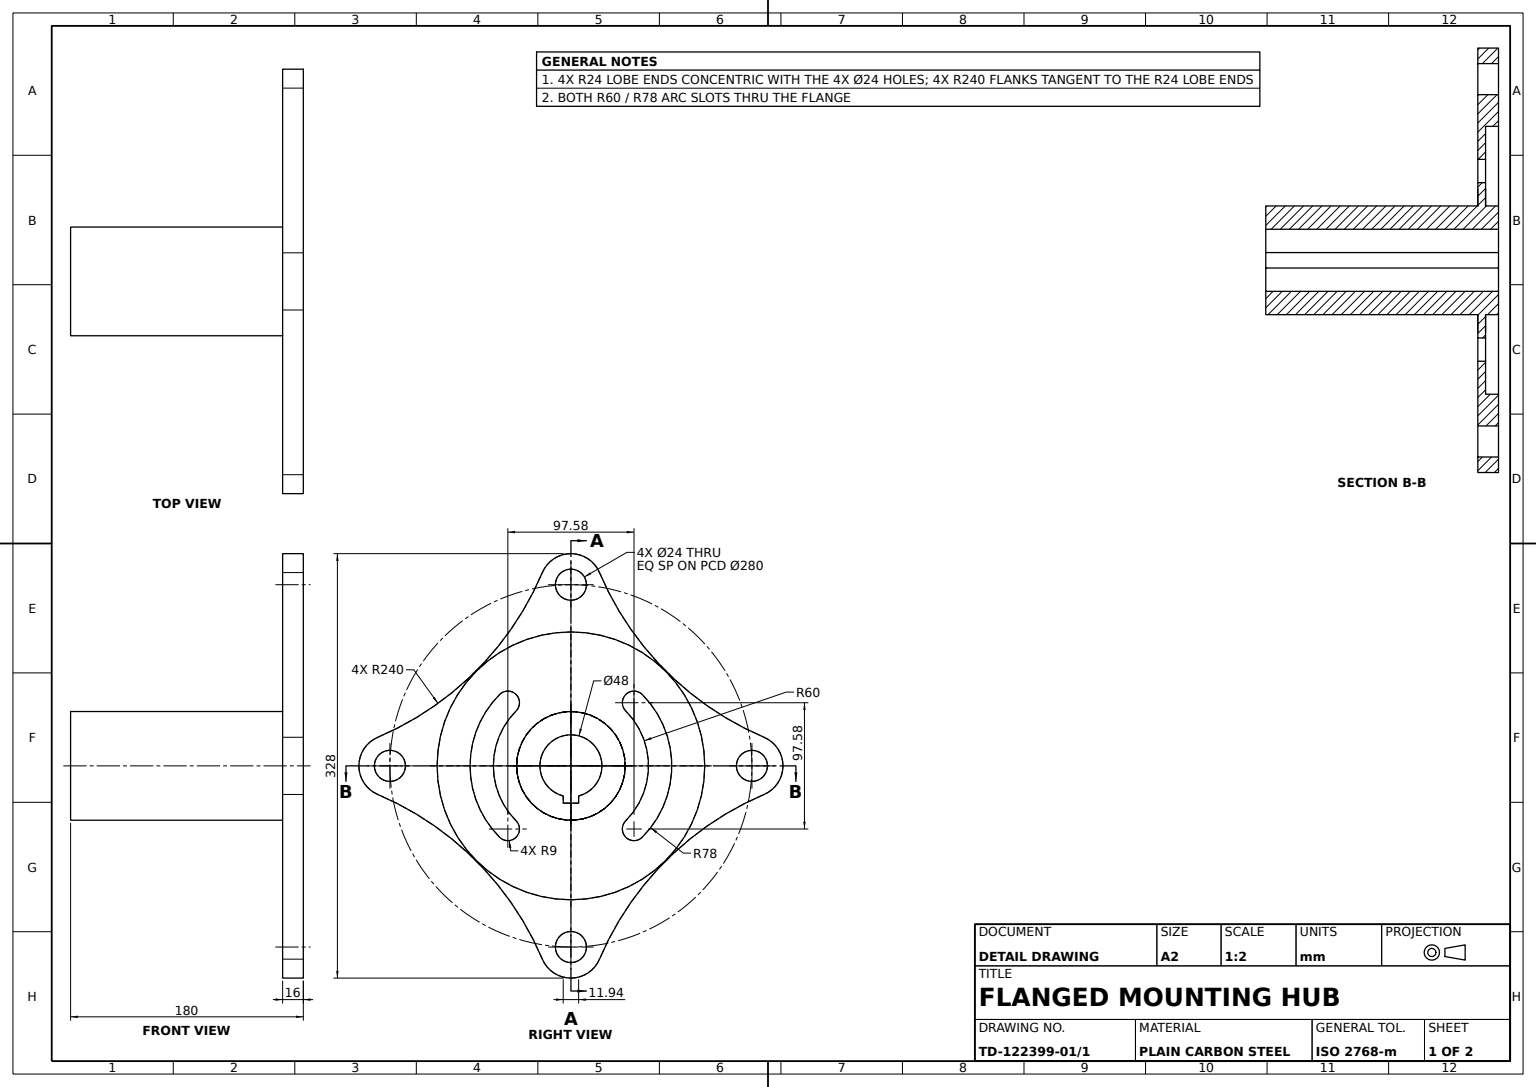
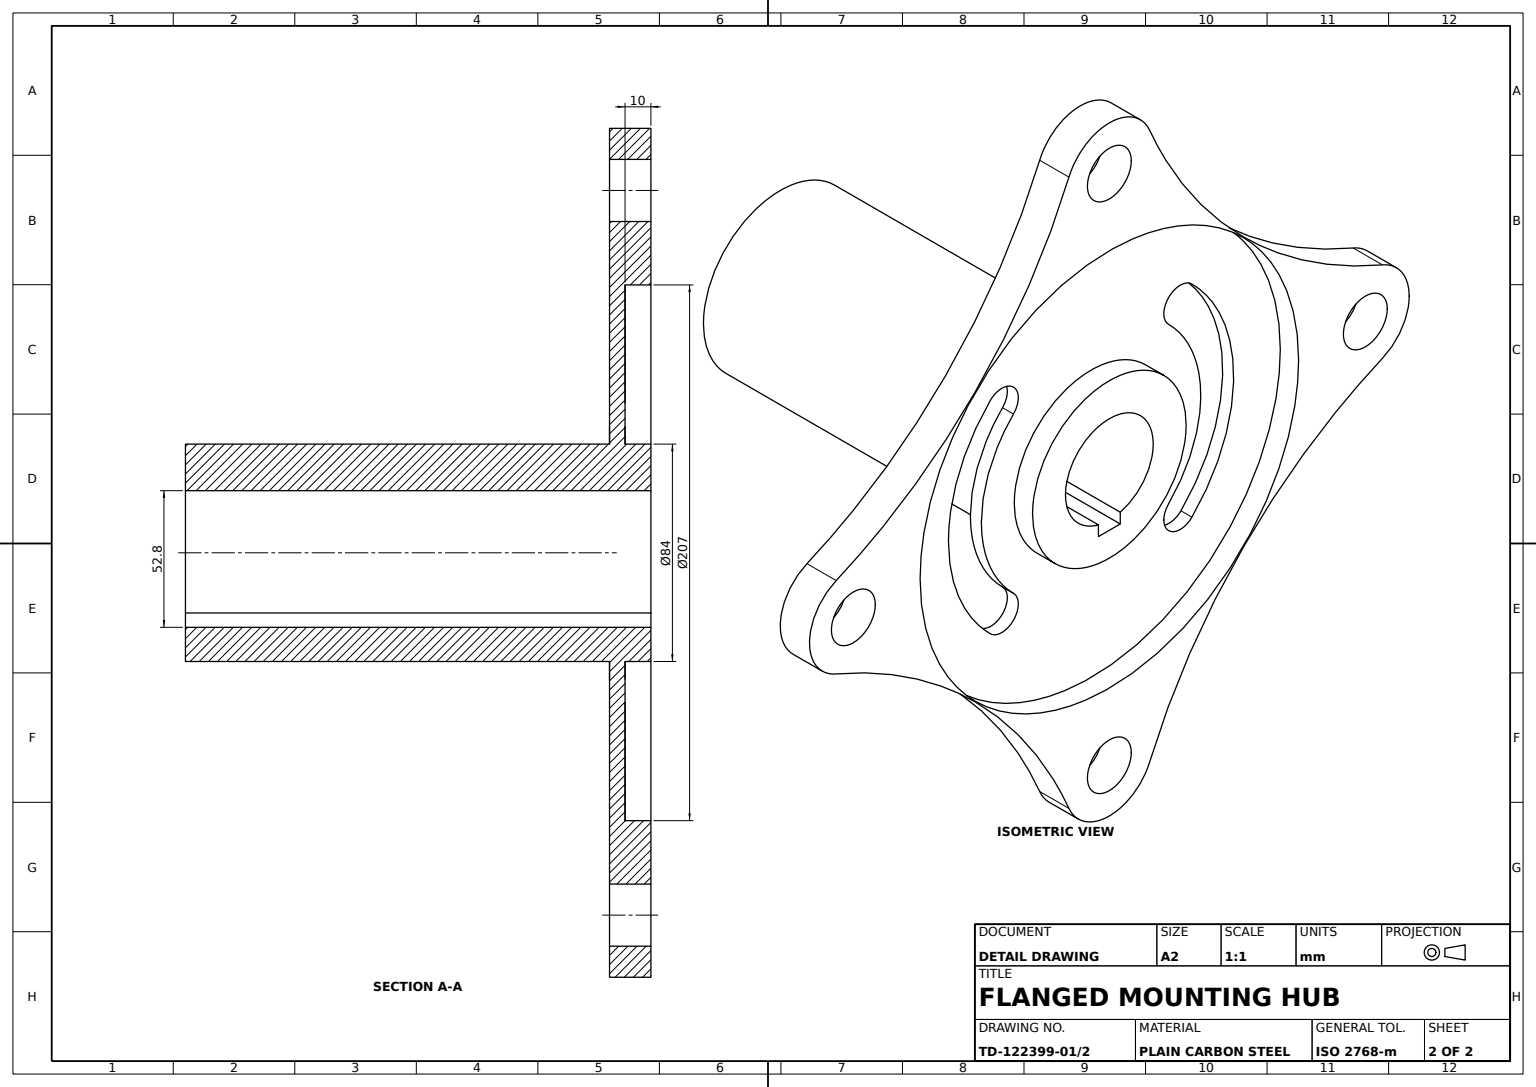
ISO-10303-21;
HEADER;
FILE_DESCRIPTION((''),'2;1');
FILE_NAME('','',(''),(''),'','','');
FILE_SCHEMA(('AUTOMOTIVE_DESIGN'));
ENDSEC;
DATA;
#1=APPLICATION_CONTEXT('');
#2=PRODUCT_CONTEXT('',#1,'mechanical');
#3=PRODUCT('','','',(#2));
#4=PRODUCT_DEFINITION_FORMATION('','',#3);
#5=PRODUCT_DEFINITION_CONTEXT('',#1,'design');
#6=PRODUCT_DEFINITION('','',#4,#5);
#7=PRODUCT_DEFINITION_SHAPE('','',#6);
#8=(LENGTH_UNIT()NAMED_UNIT(*)SI_UNIT(.MILLI.,.METRE.));
#9=(NAMED_UNIT(*)PLANE_ANGLE_UNIT()SI_UNIT($,.RADIAN.));
#10=(NAMED_UNIT(*)SI_UNIT($,.STERADIAN.)SOLID_ANGLE_UNIT());
#11=UNCERTAINTY_MEASURE_WITH_UNIT(LENGTH_MEASURE(1.E-05),#8,'distance_accuracy_value','');
#12=(GEOMETRIC_REPRESENTATION_CONTEXT(3)GLOBAL_UNCERTAINTY_ASSIGNED_CONTEXT((#11))GLOBAL_UNIT_ASSIGNED_CONTEXT((#8,#9,#10))REPRESENTATION_CONTEXT('',''));
#13=CARTESIAN_POINT('',(0.,16.,-128.));
#14=VERTEX_POINT('',#13);
#15=CARTESIAN_POINT('',(0.,0.,-128.));
#16=VERTEX_POINT('',#15);
#17=DIRECTION('',(0.,-1.,0.));
#18=VECTOR('',#17,1000.);
#19=LINE('',#13,#18);
#20=EDGE_CURVE('',#14,#16,#19,.T.);
#21=ORIENTED_EDGE('',*,*,#20,.F.);
#22=CARTESIAN_POINT('',(0.,16.,-152.));
#23=VERTEX_POINT('',#22);
#24=CARTESIAN_POINT('',(0.,16.,-140.));
#25=DIRECTION('',(0.,1.,0.));
#26=DIRECTION('',(0.,0.,1.));
#27=AXIS2_PLACEMENT_3D('',#24,#25,#26);
#28=CIRCLE('',#27,12.);
#29=EDGE_CURVE('',#14,#23,#28,.T.);
#30=ORIENTED_EDGE('',*,*,#29,.T.);
#31=CARTESIAN_POINT('',(0.,0.,-152.));
#32=VERTEX_POINT('',#31);
#33=LINE('',#22,#18);
#34=EDGE_CURVE('',#23,#32,#33,.T.);
#35=ORIENTED_EDGE('',*,*,#34,.T.);
#36=CARTESIAN_POINT('',(0.,0.,-140.));
#37=AXIS2_PLACEMENT_3D('',#36,#25,#26);
#38=CIRCLE('',#37,12.);
#39=EDGE_CURVE('',#16,#32,#38,.T.);
#40=ORIENTED_EDGE('',*,*,#39,.F.);
#41=EDGE_LOOP('',(#21,#30,#35,#40));
#42=FACE_OUTER_BOUND('',#41,.T.);
#43=DIRECTION('',(0.,0.,-1.));
#44=AXIS2_PLACEMENT_3D('',#24,#17,#43);
#45=CYLINDRICAL_SURFACE('',#44,12.);
#46=ADVANCED_FACE('',(#42),#45,.F.);
#47=CARTESIAN_POINT('',(0.,16.,-42.));
#48=VERTEX_POINT('',#47);
#49=CARTESIAN_POINT('',(0.,16.,42.));
#50=VERTEX_POINT('',#49);
#51=CARTESIAN_POINT('',(0.,16.,0.));
#52=AXIS2_PLACEMENT_3D('',#51,#25,#26);
#53=CIRCLE('',#52,42.);
#54=EDGE_CURVE('',#48,#50,#53,.T.);
#55=ORIENTED_EDGE('',*,*,#54,.T.);
#56=EDGE_CURVE('',#50,#48,#53,.T.);
#57=ORIENTED_EDGE('',*,*,#56,.T.);
#58=EDGE_LOOP('',(#55,#57));
#59=FACE_OUTER_BOUND('',#58,.T.);
#60=CARTESIAN_POINT('',(28.795625,16.,-5.97));
#61=VERTEX_POINT('',#60);
#62=CARTESIAN_POINT('',(23.245625,16.,-5.97));
#63=VERTEX_POINT('',#62);
#64=DIRECTION('',(-1.,0.,0.));
#65=VECTOR('',#64,1000.);
#66=LINE('',#62,#65);
#67=EDGE_CURVE('',#61,#63,#66,.T.);
#68=ORIENTED_EDGE('',*,*,#67,.F.);
#69=CARTESIAN_POINT('',(28.795625,16.,5.97));
#70=VERTEX_POINT('',#69);
#71=VECTOR('',#43,1000.);
#72=LINE('',#60,#71);
#73=EDGE_CURVE('',#70,#61,#72,.T.);
#74=ORIENTED_EDGE('',*,*,#73,.F.);
#75=CARTESIAN_POINT('',(23.245625,16.,5.97));
#76=VERTEX_POINT('',#75);
#77=DIRECTION('',(1.,0.,0.));
#78=VECTOR('',#77,1000.);
#79=LINE('',#75,#78);
#80=EDGE_CURVE('',#76,#70,#79,.T.);
#81=ORIENTED_EDGE('',*,*,#80,.F.);
#82=CARTESIAN_POINT('',(0.,16.,24.));
#83=VERTEX_POINT('',#82);
#84=CIRCLE('',#52,24.);
#85=EDGE_CURVE('',#83,#76,#84,.T.);
#86=ORIENTED_EDGE('',*,*,#85,.F.);
#87=CARTESIAN_POINT('',(0.,16.,-24.));
#88=VERTEX_POINT('',#87);
#89=EDGE_CURVE('',#88,#83,#84,.T.);
#90=ORIENTED_EDGE('',*,*,#89,.F.);
#91=EDGE_CURVE('',#63,#88,#84,.T.);
#92=ORIENTED_EDGE('',*,*,#91,.F.);
#93=EDGE_LOOP('',(#68,#74,#81,#86,#90,#92));
#94=FACE_BOUND('',#93,.T.);
#95=PLANE('',#52);
#96=ADVANCED_FACE('',(#59,#94),#95,.T.);
#97=CARTESIAN_POINT('',(149.368628,16.,-22.0959));
#98=VERTEX_POINT('',#97);
#99=CARTESIAN_POINT('',(22.0959,16.,-149.368628));
#100=VERTEX_POINT('',#99);
#101=CARTESIAN_POINT('',(243.054905,16.,-243.054905));
#102=AXIS2_PLACEMENT_3D('',#101,#17,#43);
#103=CIRCLE('',#102,240.);
#104=EDGE_CURVE('',#98,#100,#103,.T.);
#105=ORIENTED_EDGE('',*,*,#104,.F.);
#106=CARTESIAN_POINT('',(149.368628,0.,-22.0959));
#107=VERTEX_POINT('',#106);
#108=LINE('',#97,#18);
#109=EDGE_CURVE('',#98,#107,#108,.T.);
#110=ORIENTED_EDGE('',*,*,#109,.T.);
#111=CARTESIAN_POINT('',(22.0959,0.,-149.368628));
#112=VERTEX_POINT('',#111);
#113=CARTESIAN_POINT('',(243.054905,0.,-243.054905));
#114=AXIS2_PLACEMENT_3D('',#113,#17,#43);
#115=CIRCLE('',#114,240.);
#116=EDGE_CURVE('',#107,#112,#115,.T.);
#117=ORIENTED_EDGE('',*,*,#116,.T.);
#118=LINE('',#99,#18);
#119=EDGE_CURVE('',#100,#112,#118,.T.);
#120=ORIENTED_EDGE('',*,*,#119,.F.);
#121=EDGE_LOOP('',(#105,#110,#117,#120));
#122=FACE_OUTER_BOUND('',#121,.T.);
#123=CYLINDRICAL_SURFACE('',#102,240.);
#124=ADVANCED_FACE('',(#122),#123,.F.);
#125=CARTESIAN_POINT('',(-140.,16.,12.));
#126=VERTEX_POINT('',#125);
#127=CARTESIAN_POINT('',(-140.,0.,12.));
#128=VERTEX_POINT('',#127);
#129=LINE('',#125,#18);
#130=EDGE_CURVE('',#126,#128,#129,.T.);
#131=ORIENTED_EDGE('',*,*,#130,.F.);
#132=CARTESIAN_POINT('',(-140.,16.,-12.));
#133=VERTEX_POINT('',#132);
#134=CARTESIAN_POINT('',(-140.,16.,0.));
#135=AXIS2_PLACEMENT_3D('',#134,#25,#26);
#136=CIRCLE('',#135,12.);
#137=EDGE_CURVE('',#126,#133,#136,.T.);
#138=ORIENTED_EDGE('',*,*,#137,.T.);
#139=CARTESIAN_POINT('',(-140.,0.,-12.));
#140=VERTEX_POINT('',#139);
#141=LINE('',#132,#18);
#142=EDGE_CURVE('',#133,#140,#141,.T.);
#143=ORIENTED_EDGE('',*,*,#142,.T.);
#144=CARTESIAN_POINT('',(-140.,0.,0.));
#145=AXIS2_PLACEMENT_3D('',#144,#25,#26);
#146=CIRCLE('',#145,12.);
#147=EDGE_CURVE('',#128,#140,#146,.T.);
#148=ORIENTED_EDGE('',*,*,#147,.F.);
#149=EDGE_LOOP('',(#131,#138,#143,#148));
#150=FACE_OUTER_BOUND('',#149,.T.);
#151=AXIS2_PLACEMENT_3D('',#134,#17,#43);
#152=CYLINDRICAL_SURFACE('',#151,12.);
#153=ADVANCED_FACE('',(#150),#152,.F.);
#154=CARTESIAN_POINT('',(23.245625,-164.,5.97));
#155=VERTEX_POINT('',#154);
#156=VECTOR('',#25,1000.);
#157=LINE('',#154,#156);
#158=EDGE_CURVE('',#155,#76,#157,.T.);
#159=ORIENTED_EDGE('',*,*,#158,.T.);
#160=ORIENTED_EDGE('',*,*,#80,.T.);
#161=CARTESIAN_POINT('',(28.795625,-164.,5.97));
#162=VERTEX_POINT('',#161);
#163=LINE('',#161,#156);
#164=EDGE_CURVE('',#162,#70,#163,.T.);
#165=ORIENTED_EDGE('',*,*,#164,.F.);
#166=LINE('',#154,#78);
#167=EDGE_CURVE('',#155,#162,#166,.T.);
#168=ORIENTED_EDGE('',*,*,#167,.F.);
#169=EDGE_LOOP('',(#159,#160,#165,#168));
#170=FACE_OUTER_BOUND('',#169,.T.);
#171=AXIS2_PLACEMENT_3D('',#154,#26,#77);
#172=PLANE('',#171);
#173=ADVANCED_FACE('',(#170),#172,.F.);
#174=CARTESIAN_POINT('',(0.,6.,103.5));
#175=VERTEX_POINT('',#174);
#176=CARTESIAN_POINT('',(0.,6.,-103.5));
#177=VERTEX_POINT('',#176);
#178=CARTESIAN_POINT('',(0.,6.,0.));
#179=AXIS2_PLACEMENT_3D('',#178,#25,#26);
#180=CIRCLE('',#179,103.5);
#181=EDGE_CURVE('',#175,#177,#180,.T.);
#182=ORIENTED_EDGE('',*,*,#181,.F.);
#183=CARTESIAN_POINT('',(0.,16.,103.5));
#184=VERTEX_POINT('',#183);
#185=LINE('',#174,#156);
#186=EDGE_CURVE('',#175,#184,#185,.T.);
#187=ORIENTED_EDGE('',*,*,#186,.T.);
#188=CARTESIAN_POINT('',(0.,16.,-103.5));
#189=VERTEX_POINT('',#188);
#190=CIRCLE('',#52,103.5);
#191=EDGE_CURVE('',#184,#189,#190,.T.);
#192=ORIENTED_EDGE('',*,*,#191,.T.);
#193=LINE('',#176,#156);
#194=EDGE_CURVE('',#177,#189,#193,.T.);
#195=ORIENTED_EDGE('',*,*,#194,.F.);
#196=EDGE_LOOP('',(#182,#187,#192,#195));
#197=FACE_OUTER_BOUND('',#196,.T.);
#198=CYLINDRICAL_SURFACE('',#179,103.5);
#199=ADVANCED_FACE('',(#197),#198,.F.);
#200=CARTESIAN_POINT('',(0.,16.,128.));
#201=VERTEX_POINT('',#200);
#202=CARTESIAN_POINT('',(0.,16.,152.));
#203=VERTEX_POINT('',#202);
#204=CARTESIAN_POINT('',(0.,16.,140.));
#205=AXIS2_PLACEMENT_3D('',#204,#25,#26);
#206=CIRCLE('',#205,12.);
#207=EDGE_CURVE('',#201,#203,#206,.T.);
#208=ORIENTED_EDGE('',*,*,#207,.T.);
#209=CARTESIAN_POINT('',(0.,0.,152.));
#210=VERTEX_POINT('',#209);
#211=LINE('',#202,#18);
#212=EDGE_CURVE('',#203,#210,#211,.T.);
#213=ORIENTED_EDGE('',*,*,#212,.T.);
#214=CARTESIAN_POINT('',(0.,0.,128.));
#215=VERTEX_POINT('',#214);
#216=CARTESIAN_POINT('',(0.,0.,140.));
#217=AXIS2_PLACEMENT_3D('',#216,#25,#26);
#218=CIRCLE('',#217,12.);
#219=EDGE_CURVE('',#215,#210,#218,.T.);
#220=ORIENTED_EDGE('',*,*,#219,.F.);
#221=LINE('',#200,#18);
#222=EDGE_CURVE('',#201,#215,#221,.T.);
#223=ORIENTED_EDGE('',*,*,#222,.F.);
#224=EDGE_LOOP('',(#208,#213,#220,#223));
#225=FACE_OUTER_BOUND('',#224,.T.);
#226=AXIS2_PLACEMENT_3D('',#204,#17,#43);
#227=CYLINDRICAL_SURFACE('',#226,12.);
#228=ADVANCED_FACE('',(#225),#227,.F.);
#229=CARTESIAN_POINT('',(-48.790368,0.,-39.790368));
#230=VERTEX_POINT('',#229);
#231=CARTESIAN_POINT('',(-42.426407,0.,-42.426407));
#232=VERTEX_POINT('',#231);
#233=CARTESIAN_POINT('',(-48.790368,0.,-48.790368));
#234=AXIS2_PLACEMENT_3D('',#233,#25,#26);
#235=CIRCLE('',#234,9.);
#236=EDGE_CURVE('',#230,#232,#235,.T.);
#237=ORIENTED_EDGE('',*,*,#236,.F.);
#238=CARTESIAN_POINT('',(-48.790368,6.,-39.790368));
#239=VERTEX_POINT('',#238);
#240=CARTESIAN_POINT('',(-48.790368,-54.,-39.790368));
#241=LINE('',#240,#156);
#242=EDGE_CURVE('',#230,#239,#241,.T.);
#243=ORIENTED_EDGE('',*,*,#242,.T.);
#244=CARTESIAN_POINT('',(-42.426407,6.,-42.426407));
#245=VERTEX_POINT('',#244);
#246=CARTESIAN_POINT('',(-48.790368,6.,-48.790368));
#247=AXIS2_PLACEMENT_3D('',#246,#25,#26);
#248=CIRCLE('',#247,9.);
#249=EDGE_CURVE('',#239,#245,#248,.T.);
#250=ORIENTED_EDGE('',*,*,#249,.T.);
#251=CARTESIAN_POINT('',(-42.426407,-54.,-42.426407));
#252=LINE('',#251,#156);
#253=EDGE_CURVE('',#232,#245,#252,.T.);
#254=ORIENTED_EDGE('',*,*,#253,.F.);
#255=EDGE_LOOP('',(#237,#243,#250,#254));
#256=FACE_OUTER_BOUND('',#255,.T.);
#257=CARTESIAN_POINT('',(-48.790368,-54.,-48.790368));
#258=AXIS2_PLACEMENT_3D('',#257,#25,#26);
#259=CYLINDRICAL_SURFACE('',#258,9.);
#260=ADVANCED_FACE('',(#256),#259,.F.);
#261=ORIENTED_EDGE('',*,*,#34,.F.);
#262=EDGE_CURVE('',#23,#14,#28,.T.);
#263=ORIENTED_EDGE('',*,*,#262,.T.);
#264=ORIENTED_EDGE('',*,*,#20,.T.);
#265=EDGE_CURVE('',#32,#16,#38,.T.);
#266=ORIENTED_EDGE('',*,*,#265,.F.);
#267=EDGE_LOOP('',(#261,#263,#264,#266));
#268=FACE_OUTER_BOUND('',#267,.T.);
#269=ADVANCED_FACE('',(#268),#45,.F.);
#270=CARTESIAN_POINT('',(0.,6.,-42.));
#271=VERTEX_POINT('',#270);
#272=CARTESIAN_POINT('',(0.,6.,42.));
#273=VERTEX_POINT('',#272);
#274=CIRCLE('',#179,42.);
#275=EDGE_CURVE('',#271,#273,#274,.T.);
#276=ORIENTED_EDGE('',*,*,#275,.T.);
#277=CARTESIAN_POINT('',(0.,-164.,42.));
#278=LINE('',#277,#156);
#279=EDGE_CURVE('',#273,#50,#278,.T.);
#280=ORIENTED_EDGE('',*,*,#279,.T.);
#281=ORIENTED_EDGE('',*,*,#54,.F.);
#282=CARTESIAN_POINT('',(0.,-164.,-42.));
#283=LINE('',#282,#156);
#284=EDGE_CURVE('',#271,#48,#283,.T.);
#285=ORIENTED_EDGE('',*,*,#284,.F.);
#286=EDGE_LOOP('',(#276,#280,#281,#285));
#287=FACE_OUTER_BOUND('',#286,.T.);
#288=CARTESIAN_POINT('',(0.,-164.,0.));
#289=AXIS2_PLACEMENT_3D('',#288,#25,#26);
#290=CYLINDRICAL_SURFACE('',#289,42.);
#291=ADVANCED_FACE('',(#287),#290,.T.);
#292=CARTESIAN_POINT('',(0.,6.,60.));
#293=VERTEX_POINT('',#292);
#294=CARTESIAN_POINT('',(-42.426407,6.,42.426407));
#295=VERTEX_POINT('',#294);
#296=AXIS2_PLACEMENT_3D('',#178,#17,#43);
#297=CIRCLE('',#296,60.);
#298=EDGE_CURVE('',#293,#295,#297,.T.);
#299=ORIENTED_EDGE('',*,*,#298,.T.);
#300=CARTESIAN_POINT('',(-42.426407,0.,42.426407));
#301=VERTEX_POINT('',#300);
#302=CARTESIAN_POINT('',(-42.426407,-54.,42.426407));
#303=LINE('',#302,#156);
#304=EDGE_CURVE('',#301,#295,#303,.T.);
#305=ORIENTED_EDGE('',*,*,#304,.F.);
#306=CARTESIAN_POINT('',(0.,0.,60.));
#307=VERTEX_POINT('',#306);
#308=CARTESIAN_POINT('',(0.,0.,0.));
#309=AXIS2_PLACEMENT_3D('',#308,#17,#26);
#310=CIRCLE('',#309,60.);
#311=EDGE_CURVE('',#307,#301,#310,.T.);
#312=ORIENTED_EDGE('',*,*,#311,.F.);
#313=CARTESIAN_POINT('',(0.,-54.,60.));
#314=LINE('',#313,#156);
#315=EDGE_CURVE('',#307,#293,#314,.T.);
#316=ORIENTED_EDGE('',*,*,#315,.T.);
#317=EDGE_LOOP('',(#299,#305,#312,#316));
#318=FACE_OUTER_BOUND('',#317,.T.);
#319=CARTESIAN_POINT('',(0.,-54.,0.));
#320=AXIS2_PLACEMENT_3D('',#319,#25,#26);
#321=CYLINDRICAL_SURFACE('',#320,60.);
#322=ADVANCED_FACE('',(#318),#321,.T.);
#323=CARTESIAN_POINT('',(28.795625,-164.,-5.97));
#324=VERTEX_POINT('',#323);
#325=LINE('',#323,#156);
#326=EDGE_CURVE('',#324,#61,#325,.T.);
#327=ORIENTED_EDGE('',*,*,#326,.F.);
#328=LINE('',#323,#71);
#329=EDGE_CURVE('',#162,#324,#328,.T.);
#330=ORIENTED_EDGE('',*,*,#329,.F.);
#331=ORIENTED_EDGE('',*,*,#164,.T.);
#332=ORIENTED_EDGE('',*,*,#73,.T.);
#333=EDGE_LOOP('',(#327,#330,#331,#332));
#334=FACE_OUTER_BOUND('',#333,.T.);
#335=AXIS2_PLACEMENT_3D('',#323,#77,#43);
#336=PLANE('',#335);
#337=ADVANCED_FACE('',(#334),#336,.F.);
#338=CARTESIAN_POINT('',(-55.154329,0.,-55.154329));
#339=VERTEX_POINT('',#338);
#340=EDGE_CURVE('',#339,#230,#235,.T.);
#341=ORIENTED_EDGE('',*,*,#340,.F.);
#342=CARTESIAN_POINT('',(-55.154329,6.,-55.154329));
#343=VERTEX_POINT('',#342);
#344=CARTESIAN_POINT('',(-55.154329,-54.,-55.154329));
#345=LINE('',#344,#156);
#346=EDGE_CURVE('',#339,#343,#345,.T.);
#347=ORIENTED_EDGE('',*,*,#346,.T.);
#348=EDGE_CURVE('',#343,#239,#248,.T.);
#349=ORIENTED_EDGE('',*,*,#348,.T.);
#350=ORIENTED_EDGE('',*,*,#242,.F.);
#351=EDGE_LOOP('',(#341,#347,#349,#350));
#352=FACE_OUTER_BOUND('',#351,.T.);
#353=ADVANCED_FACE('',(#352),#259,.F.);
#354=ORIENTED_EDGE('',*,*,#119,.T.);
#355=CARTESIAN_POINT('',(0.,0.,-164.));
#356=VERTEX_POINT('',#355);
#357=CIRCLE('',#37,24.);
#358=EDGE_CURVE('',#112,#356,#357,.T.);
#359=ORIENTED_EDGE('',*,*,#358,.T.);
#360=CARTESIAN_POINT('',(0.,16.,-164.));
#361=VERTEX_POINT('',#360);
#362=LINE('',#360,#18);
#363=EDGE_CURVE('',#361,#356,#362,.T.);
#364=ORIENTED_EDGE('',*,*,#363,.F.);
#365=CIRCLE('',#27,24.);
#366=EDGE_CURVE('',#100,#361,#365,.T.);
#367=ORIENTED_EDGE('',*,*,#366,.F.);
#368=EDGE_LOOP('',(#354,#359,#364,#367));
#369=FACE_OUTER_BOUND('',#368,.T.);
#370=CYLINDRICAL_SURFACE('',#44,24.);
#371=ADVANCED_FACE('',(#369),#370,.T.);
#372=CARTESIAN_POINT('',(42.426407,0.,42.426407));
#373=VERTEX_POINT('',#372);
#374=CARTESIAN_POINT('',(42.426407,6.,42.426407));
#375=VERTEX_POINT('',#374);
#376=CARTESIAN_POINT('',(42.426407,-54.,42.426407));
#377=LINE('',#376,#156);
#378=EDGE_CURVE('',#373,#375,#377,.T.);
#379=ORIENTED_EDGE('',*,*,#378,.F.);
#380=CARTESIAN_POINT('',(55.154329,0.,55.154329));
#381=VERTEX_POINT('',#380);
#382=CARTESIAN_POINT('',(48.790368,0.,48.790368));
#383=AXIS2_PLACEMENT_3D('',#382,#25,#26);
#384=CIRCLE('',#383,9.);
#385=EDGE_CURVE('',#381,#373,#384,.T.);
#386=ORIENTED_EDGE('',*,*,#385,.F.);
#387=CARTESIAN_POINT('',(55.154329,6.,55.154329));
#388=VERTEX_POINT('',#387);
#389=CARTESIAN_POINT('',(55.154329,-54.,55.154329));
#390=LINE('',#389,#156);
#391=EDGE_CURVE('',#381,#388,#390,.T.);
#392=ORIENTED_EDGE('',*,*,#391,.T.);
#393=CARTESIAN_POINT('',(48.790368,6.,48.790368));
#394=AXIS2_PLACEMENT_3D('',#393,#25,#43);
#395=CIRCLE('',#394,9.);
#396=EDGE_CURVE('',#388,#375,#395,.T.);
#397=ORIENTED_EDGE('',*,*,#396,.T.);
#398=EDGE_LOOP('',(#379,#386,#392,#397));
#399=FACE_OUTER_BOUND('',#398,.T.);
#400=CARTESIAN_POINT('',(48.790368,-54.,48.790368));
#401=AXIS2_PLACEMENT_3D('',#400,#25,#26);
#402=CYLINDRICAL_SURFACE('',#401,9.);
#403=ADVANCED_FACE('',(#399),#402,.F.);
#404=CARTESIAN_POINT('',(-149.368628,16.,22.0959));
#405=VERTEX_POINT('',#404);
#406=CARTESIAN_POINT('',(-149.368628,0.,22.0959));
#407=VERTEX_POINT('',#406);
#408=LINE('',#404,#18);
#409=EDGE_CURVE('',#405,#407,#408,.T.);
#410=ORIENTED_EDGE('',*,*,#409,.F.);
#411=CARTESIAN_POINT('',(-149.368628,16.,-22.0959));
#412=VERTEX_POINT('',#411);
#413=CIRCLE('',#135,24.);
#414=EDGE_CURVE('',#412,#405,#413,.T.);
#415=ORIENTED_EDGE('',*,*,#414,.F.);
#416=CARTESIAN_POINT('',(-149.368628,0.,-22.0959));
#417=VERTEX_POINT('',#416);
#418=LINE('',#411,#18);
#419=EDGE_CURVE('',#412,#417,#418,.T.);
#420=ORIENTED_EDGE('',*,*,#419,.T.);
#421=CIRCLE('',#145,24.);
#422=EDGE_CURVE('',#417,#407,#421,.T.);
#423=ORIENTED_EDGE('',*,*,#422,.T.);
#424=EDGE_LOOP('',(#410,#415,#420,#423));
#425=FACE_OUTER_BOUND('',#424,.T.);
#426=CYLINDRICAL_SURFACE('',#151,24.);
#427=ADVANCED_FACE('',(#425),#426,.T.);
#428=CARTESIAN_POINT('',(-22.0959,16.,-149.368628));
#429=VERTEX_POINT('',#428);
#430=CARTESIAN_POINT('',(-22.0959,0.,-149.368628));
#431=VERTEX_POINT('',#430);
#432=LINE('',#428,#18);
#433=EDGE_CURVE('',#429,#431,#432,.T.);
#434=ORIENTED_EDGE('',*,*,#433,.T.);
#435=CARTESIAN_POINT('',(-243.054905,0.,-243.054905));
#436=AXIS2_PLACEMENT_3D('',#435,#17,#26);
#437=CIRCLE('',#436,240.);
#438=EDGE_CURVE('',#431,#417,#437,.T.);
#439=ORIENTED_EDGE('',*,*,#438,.T.);
#440=ORIENTED_EDGE('',*,*,#419,.F.);
#441=CARTESIAN_POINT('',(-243.054905,16.,-243.054905));
#442=AXIS2_PLACEMENT_3D('',#441,#17,#26);
#443=CIRCLE('',#442,240.);
#444=EDGE_CURVE('',#429,#412,#443,.T.);
#445=ORIENTED_EDGE('',*,*,#444,.F.);
#446=EDGE_LOOP('',(#434,#439,#440,#445));
#447=FACE_OUTER_BOUND('',#446,.T.);
#448=AXIS2_PLACEMENT_3D('',#441,#17,#43);
#449=CYLINDRICAL_SURFACE('',#448,240.);
#450=ADVANCED_FACE('',(#447),#449,.F.);
#451=CARTESIAN_POINT('',(0.,6.,78.));
#452=VERTEX_POINT('',#451);
#453=AXIS2_PLACEMENT_3D('',#178,#25,#43);
#454=CIRCLE('',#453,78.);
#455=EDGE_CURVE('',#452,#388,#454,.T.);
#456=ORIENTED_EDGE('',*,*,#455,.T.);
#457=ORIENTED_EDGE('',*,*,#391,.F.);
#458=CARTESIAN_POINT('',(0.,0.,78.));
#459=VERTEX_POINT('',#458);
#460=AXIS2_PLACEMENT_3D('',#308,#25,#26);
#461=CIRCLE('',#460,78.);
#462=EDGE_CURVE('',#459,#381,#461,.T.);
#463=ORIENTED_EDGE('',*,*,#462,.F.);
#464=CARTESIAN_POINT('',(0.,-54.,78.));
#465=LINE('',#464,#156);
#466=EDGE_CURVE('',#459,#452,#465,.T.);
#467=ORIENTED_EDGE('',*,*,#466,.T.);
#468=EDGE_LOOP('',(#456,#457,#463,#467));
#469=FACE_OUTER_BOUND('',#468,.T.);
#470=CYLINDRICAL_SURFACE('',#320,78.);
#471=ADVANCED_FACE('',(#469),#470,.F.);
#472=CARTESIAN_POINT('',(149.368628,16.,22.0959));
#473=VERTEX_POINT('',#472);
#474=CARTESIAN_POINT('',(140.,16.,0.));
#475=AXIS2_PLACEMENT_3D('',#474,#25,#26);
#476=CIRCLE('',#475,24.);
#477=EDGE_CURVE('',#473,#98,#476,.T.);
#478=ORIENTED_EDGE('',*,*,#477,.F.);
#479=CARTESIAN_POINT('',(149.368628,0.,22.0959));
#480=VERTEX_POINT('',#479);
#481=LINE('',#472,#18);
#482=EDGE_CURVE('',#473,#480,#481,.T.);
#483=ORIENTED_EDGE('',*,*,#482,.T.);
#484=CARTESIAN_POINT('',(140.,0.,0.));
#485=AXIS2_PLACEMENT_3D('',#484,#25,#26);
#486=CIRCLE('',#485,24.);
#487=EDGE_CURVE('',#480,#107,#486,.T.);
#488=ORIENTED_EDGE('',*,*,#487,.T.);
#489=ORIENTED_EDGE('',*,*,#109,.F.);
#490=EDGE_LOOP('',(#478,#483,#488,#489));
#491=FACE_OUTER_BOUND('',#490,.T.);
#492=AXIS2_PLACEMENT_3D('',#474,#17,#43);
#493=CYLINDRICAL_SURFACE('',#492,24.);
#494=ADVANCED_FACE('',(#491),#493,.T.);
#495=EDGE_CURVE('',#140,#128,#146,.T.);
#496=ORIENTED_EDGE('',*,*,#495,.F.);
#497=ORIENTED_EDGE('',*,*,#142,.F.);
#498=EDGE_CURVE('',#133,#126,#136,.T.);
#499=ORIENTED_EDGE('',*,*,#498,.T.);
#500=ORIENTED_EDGE('',*,*,#130,.T.);
#501=EDGE_LOOP('',(#496,#497,#499,#500));
#502=FACE_OUTER_BOUND('',#501,.T.);
#503=ADVANCED_FACE('',(#502),#152,.F.);
#504=CARTESIAN_POINT('',(42.426407,6.,-42.426407));
#505=VERTEX_POINT('',#504);
#506=AXIS2_PLACEMENT_3D('',#178,#17,#26);
#507=CIRCLE('',#506,60.);
#508=EDGE_CURVE('',#245,#505,#507,.T.);
#509=ORIENTED_EDGE('',*,*,#508,.T.);
#510=CARTESIAN_POINT('',(42.426407,0.,-42.426407));
#511=VERTEX_POINT('',#510);
#512=CARTESIAN_POINT('',(42.426407,-54.,-42.426407));
#513=LINE('',#512,#156);
#514=EDGE_CURVE('',#511,#505,#513,.T.);
#515=ORIENTED_EDGE('',*,*,#514,.F.);
#516=EDGE_CURVE('',#232,#511,#310,.T.);
#517=ORIENTED_EDGE('',*,*,#516,.F.);
#518=ORIENTED_EDGE('',*,*,#253,.T.);
#519=EDGE_LOOP('',(#509,#515,#517,#518));
#520=FACE_OUTER_BOUND('',#519,.T.);
#521=ADVANCED_FACE('',(#520),#321,.T.);
#522=ORIENTED_EDGE('',*,*,#433,.F.);
#523=EDGE_CURVE('',#361,#429,#365,.T.);
#524=ORIENTED_EDGE('',*,*,#523,.F.);
#525=ORIENTED_EDGE('',*,*,#363,.T.);
#526=EDGE_CURVE('',#356,#431,#357,.T.);
#527=ORIENTED_EDGE('',*,*,#526,.T.);
#528=EDGE_LOOP('',(#522,#524,#525,#527));
#529=FACE_OUTER_BOUND('',#528,.T.);
#530=ADVANCED_FACE('',(#529),#370,.T.);
#531=CARTESIAN_POINT('',(0.,-164.,-24.));
#532=VERTEX_POINT('',#531);
#533=LINE('',#531,#156);
#534=EDGE_CURVE('',#532,#88,#533,.T.);
#535=ORIENTED_EDGE('',*,*,#534,.F.);
#536=CARTESIAN_POINT('',(23.245625,-164.,-5.97));
#537=VERTEX_POINT('',#536);
#538=CIRCLE('',#289,24.);
#539=EDGE_CURVE('',#537,#532,#538,.T.);
#540=ORIENTED_EDGE('',*,*,#539,.F.);
#541=LINE('',#536,#156);
#542=EDGE_CURVE('',#537,#63,#541,.T.);
#543=ORIENTED_EDGE('',*,*,#542,.T.);
#544=ORIENTED_EDGE('',*,*,#91,.T.);
#545=EDGE_LOOP('',(#535,#540,#543,#544));
#546=FACE_OUTER_BOUND('',#545,.T.);
#547=CYLINDRICAL_SURFACE('',#289,24.);
#548=ADVANCED_FACE('',(#546),#547,.F.);
#549=CARTESIAN_POINT('',(-22.0959,16.,149.368628));
#550=VERTEX_POINT('',#549);
#551=CARTESIAN_POINT('',(22.0959,16.,149.368628));
#552=VERTEX_POINT('',#551);
#553=CIRCLE('',#205,24.);
#554=EDGE_CURVE('',#550,#552,#553,.T.);
#555=ORIENTED_EDGE('',*,*,#554,.F.);
#556=CARTESIAN_POINT('',(-22.0959,0.,149.368628));
#557=VERTEX_POINT('',#556);
#558=LINE('',#549,#18);
#559=EDGE_CURVE('',#550,#557,#558,.T.);
#560=ORIENTED_EDGE('',*,*,#559,.T.);
#561=CARTESIAN_POINT('',(22.0959,0.,149.368628));
#562=VERTEX_POINT('',#561);
#563=CIRCLE('',#217,24.);
#564=EDGE_CURVE('',#557,#562,#563,.T.);
#565=ORIENTED_EDGE('',*,*,#564,.T.);
#566=LINE('',#551,#18);
#567=EDGE_CURVE('',#552,#562,#566,.T.);
#568=ORIENTED_EDGE('',*,*,#567,.F.);
#569=EDGE_LOOP('',(#555,#560,#565,#568));
#570=FACE_OUTER_BOUND('',#569,.T.);
#571=CYLINDRICAL_SURFACE('',#226,24.);
#572=ADVANCED_FACE('',(#570),#571,.T.);
#573=CARTESIAN_POINT('',(140.,16.,12.));
#574=VERTEX_POINT('',#573);
#575=CARTESIAN_POINT('',(140.,16.,-12.));
#576=VERTEX_POINT('',#575);
#577=CIRCLE('',#475,12.);
#578=EDGE_CURVE('',#574,#576,#577,.T.);
#579=ORIENTED_EDGE('',*,*,#578,.F.);
#580=EDGE_CURVE('',#576,#574,#577,.T.);
#581=ORIENTED_EDGE('',*,*,#580,.F.);
#582=EDGE_LOOP('',(#579,#581));
#583=FACE_BOUND('',#582,.T.);
#584=ORIENTED_EDGE('',*,*,#29,.F.);
#585=ORIENTED_EDGE('',*,*,#262,.F.);
#586=EDGE_LOOP('',(#584,#585));
#587=FACE_BOUND('',#586,.T.);
#588=CARTESIAN_POINT('',(243.054905,16.,243.054905));
#589=AXIS2_PLACEMENT_3D('',#588,#17,#26);
#590=CIRCLE('',#589,240.);
#591=EDGE_CURVE('',#552,#473,#590,.T.);
#592=ORIENTED_EDGE('',*,*,#591,.T.);
#593=ORIENTED_EDGE('',*,*,#477,.T.);
#594=ORIENTED_EDGE('',*,*,#104,.T.);
#595=ORIENTED_EDGE('',*,*,#366,.T.);
#596=ORIENTED_EDGE('',*,*,#523,.T.);
#597=ORIENTED_EDGE('',*,*,#444,.T.);
#598=ORIENTED_EDGE('',*,*,#414,.T.);
#599=CARTESIAN_POINT('',(-243.054905,16.,243.054905));
#600=AXIS2_PLACEMENT_3D('',#599,#17,#43);
#601=CIRCLE('',#600,240.);
#602=EDGE_CURVE('',#405,#550,#601,.T.);
#603=ORIENTED_EDGE('',*,*,#602,.T.);
#604=ORIENTED_EDGE('',*,*,#554,.T.);
#605=EDGE_LOOP('',(#592,#593,#594,#595,#596,#597,#598,#603,#604));
#606=FACE_OUTER_BOUND('',#605,.T.);
#607=ORIENTED_EDGE('',*,*,#207,.F.);
#608=EDGE_CURVE('',#203,#201,#206,.T.);
#609=ORIENTED_EDGE('',*,*,#608,.F.);
#610=EDGE_LOOP('',(#607,#609));
#611=FACE_BOUND('',#610,.T.);
#612=ORIENTED_EDGE('',*,*,#498,.F.);
#613=ORIENTED_EDGE('',*,*,#137,.F.);
#614=EDGE_LOOP('',(#612,#613));
#615=FACE_BOUND('',#614,.T.);
#616=EDGE_CURVE('',#189,#184,#190,.T.);
#617=ORIENTED_EDGE('',*,*,#616,.F.);
#618=ORIENTED_EDGE('',*,*,#191,.F.);
#619=EDGE_LOOP('',(#617,#618));
#620=FACE_BOUND('',#619,.T.);
#621=CARTESIAN_POINT('',(121.527452,16.,191.527452));
#622=AXIS2_PLACEMENT_3D('',#621,#25,#26);
#623=PLANE('',#622);
#624=ADVANCED_FACE('',(#583,#587,#606,#611,#615,#620),#623,.T.);
#625=ORIENTED_EDGE('',*,*,#315,.F.);
#626=EDGE_CURVE('',#373,#307,#310,.T.);
#627=ORIENTED_EDGE('',*,*,#626,.F.);
#628=ORIENTED_EDGE('',*,*,#378,.T.);
#629=EDGE_CURVE('',#375,#293,#297,.T.);
#630=ORIENTED_EDGE('',*,*,#629,.T.);
#631=EDGE_LOOP('',(#625,#627,#628,#630));
#632=FACE_OUTER_BOUND('',#631,.T.);
#633=ADVANCED_FACE('',(#632),#321,.T.);
#634=VERTEX_POINT('',#277);
#635=CARTESIAN_POINT('',(0.,0.,42.));
#636=VERTEX_POINT('',#635);
#637=EDGE_CURVE('',#634,#636,#278,.T.);
#638=ORIENTED_EDGE('',*,*,#637,.T.);
#639=CARTESIAN_POINT('',(0.,0.,-42.));
#640=VERTEX_POINT('',#639);
#641=CIRCLE('',#460,42.);
#642=EDGE_CURVE('',#640,#636,#641,.T.);
#643=ORIENTED_EDGE('',*,*,#642,.F.);
#644=VERTEX_POINT('',#282);
#645=EDGE_CURVE('',#644,#640,#283,.T.);
#646=ORIENTED_EDGE('',*,*,#645,.F.);
#647=CIRCLE('',#289,42.);
#648=EDGE_CURVE('',#644,#634,#647,.T.);
#649=ORIENTED_EDGE('',*,*,#648,.T.);
#650=EDGE_LOOP('',(#638,#643,#646,#649));
#651=FACE_OUTER_BOUND('',#650,.T.);
#652=ADVANCED_FACE('',(#651),#290,.T.);
#653=CARTESIAN_POINT('',(140.,0.,-12.));
#654=VERTEX_POINT('',#653);
#655=CARTESIAN_POINT('',(140.,0.,12.));
#656=VERTEX_POINT('',#655);
#657=CIRCLE('',#485,12.);
#658=EDGE_CURVE('',#654,#656,#657,.T.);
#659=ORIENTED_EDGE('',*,*,#658,.T.);
#660=EDGE_CURVE('',#656,#654,#657,.T.);
#661=ORIENTED_EDGE('',*,*,#660,.T.);
#662=EDGE_LOOP('',(#659,#661));
#663=FACE_BOUND('',#662,.T.);
#664=ORIENTED_EDGE('',*,*,#116,.F.);
#665=ORIENTED_EDGE('',*,*,#487,.F.);
#666=CARTESIAN_POINT('',(243.054905,0.,243.054905));
#667=AXIS2_PLACEMENT_3D('',#666,#17,#26);
#668=CIRCLE('',#667,240.);
#669=EDGE_CURVE('',#562,#480,#668,.T.);
#670=ORIENTED_EDGE('',*,*,#669,.F.);
#671=ORIENTED_EDGE('',*,*,#564,.F.);
#672=CARTESIAN_POINT('',(-243.054905,0.,243.054905));
#673=AXIS2_PLACEMENT_3D('',#672,#17,#43);
#674=CIRCLE('',#673,240.);
#675=EDGE_CURVE('',#407,#557,#674,.T.);
#676=ORIENTED_EDGE('',*,*,#675,.F.);
#677=ORIENTED_EDGE('',*,*,#422,.F.);
#678=ORIENTED_EDGE('',*,*,#438,.F.);
#679=ORIENTED_EDGE('',*,*,#526,.F.);
#680=ORIENTED_EDGE('',*,*,#358,.F.);
#681=EDGE_LOOP('',(#664,#665,#670,#671,#676,#677,#678,#679,#680));
#682=FACE_OUTER_BOUND('',#681,.T.);
#683=ORIENTED_EDGE('',*,*,#642,.T.);
#684=EDGE_CURVE('',#636,#640,#641,.T.);
#685=ORIENTED_EDGE('',*,*,#684,.T.);
#686=EDGE_LOOP('',(#683,#685));
#687=FACE_BOUND('',#686,.T.);
#688=ORIENTED_EDGE('',*,*,#385,.T.);
#689=ORIENTED_EDGE('',*,*,#626,.T.);
#690=ORIENTED_EDGE('',*,*,#311,.T.);
#691=CARTESIAN_POINT('',(-55.154329,0.,55.154329));
#692=VERTEX_POINT('',#691);
#693=CARTESIAN_POINT('',(-48.790368,0.,48.790368));
#694=AXIS2_PLACEMENT_3D('',#693,#25,#26);
#695=CIRCLE('',#694,9.);
#696=EDGE_CURVE('',#301,#692,#695,.T.);
#697=ORIENTED_EDGE('',*,*,#696,.T.);
#698=EDGE_CURVE('',#692,#459,#461,.T.);
#699=ORIENTED_EDGE('',*,*,#698,.T.);
#700=ORIENTED_EDGE('',*,*,#462,.T.);
#701=EDGE_LOOP('',(#688,#689,#690,#697,#699,#700));
#702=FACE_BOUND('',#701,.T.);
#703=ORIENTED_EDGE('',*,*,#39,.T.);
#704=ORIENTED_EDGE('',*,*,#265,.T.);
#705=EDGE_LOOP('',(#703,#704));
#706=FACE_BOUND('',#705,.T.);
#707=ORIENTED_EDGE('',*,*,#495,.T.);
#708=ORIENTED_EDGE('',*,*,#147,.T.);
#709=EDGE_LOOP('',(#707,#708));
#710=FACE_BOUND('',#709,.T.);
#711=ORIENTED_EDGE('',*,*,#219,.T.);
#712=EDGE_CURVE('',#210,#215,#218,.T.);
#713=ORIENTED_EDGE('',*,*,#712,.T.);
#714=EDGE_LOOP('',(#711,#713));
#715=FACE_BOUND('',#714,.T.);
#716=CARTESIAN_POINT('',(48.790368,0.,-39.790368));
#717=VERTEX_POINT('',#716);
#718=CARTESIAN_POINT('',(55.154329,0.,-55.154329));
#719=VERTEX_POINT('',#718);
#720=CARTESIAN_POINT('',(48.790368,0.,-48.790368));
#721=AXIS2_PLACEMENT_3D('',#720,#25,#26);
#722=CIRCLE('',#721,9.);
#723=EDGE_CURVE('',#717,#719,#722,.T.);
#724=ORIENTED_EDGE('',*,*,#723,.T.);
#725=EDGE_CURVE('',#719,#339,#461,.T.);
#726=ORIENTED_EDGE('',*,*,#725,.T.);
#727=ORIENTED_EDGE('',*,*,#340,.T.);
#728=ORIENTED_EDGE('',*,*,#236,.T.);
#729=ORIENTED_EDGE('',*,*,#516,.T.);
#730=EDGE_CURVE('',#511,#717,#722,.T.);
#731=ORIENTED_EDGE('',*,*,#730,.T.);
#732=EDGE_LOOP('',(#724,#726,#727,#728,#729,#731));
#733=FACE_BOUND('',#732,.T.);
#734=CARTESIAN_POINT('',(121.527452,0.,191.527452));
#735=AXIS2_PLACEMENT_3D('',#734,#25,#26);
#736=PLANE('',#735);
#737=ADVANCED_FACE('',(#663,#682,#687,#702,#706,#710,#715,#733),#736,.F.);
#738=ORIENTED_EDGE('',*,*,#542,.F.);
#739=LINE('',#536,#65);
#740=EDGE_CURVE('',#324,#537,#739,.T.);
#741=ORIENTED_EDGE('',*,*,#740,.F.);
#742=ORIENTED_EDGE('',*,*,#326,.T.);
#743=ORIENTED_EDGE('',*,*,#67,.T.);
#744=EDGE_LOOP('',(#738,#741,#742,#743));
#745=FACE_OUTER_BOUND('',#744,.T.);
#746=AXIS2_PLACEMENT_3D('',#536,#43,#64);
#747=PLANE('',#746);
#748=ADVANCED_FACE('',(#745),#747,.F.);
#749=CARTESIAN_POINT('',(-55.154329,6.,55.154329));
#750=VERTEX_POINT('',#749);
#751=CARTESIAN_POINT('',(-55.154329,-54.,55.154329));
#752=LINE('',#751,#156);
#753=EDGE_CURVE('',#692,#750,#752,.T.);
#754=ORIENTED_EDGE('',*,*,#753,.F.);
#755=ORIENTED_EDGE('',*,*,#696,.F.);
#756=ORIENTED_EDGE('',*,*,#304,.T.);
#757=CARTESIAN_POINT('',(-48.790368,6.,48.790368));
#758=AXIS2_PLACEMENT_3D('',#757,#25,#43);
#759=CIRCLE('',#758,9.);
#760=EDGE_CURVE('',#295,#750,#759,.T.);
#761=ORIENTED_EDGE('',*,*,#760,.T.);
#762=EDGE_LOOP('',(#754,#755,#756,#761));
#763=FACE_OUTER_BOUND('',#762,.T.);
#764=CARTESIAN_POINT('',(-48.790368,-54.,48.790368));
#765=AXIS2_PLACEMENT_3D('',#764,#25,#26);
#766=CYLINDRICAL_SURFACE('',#765,9.);
#767=ADVANCED_FACE('',(#763),#766,.F.);
#768=LINE('',#575,#18);
#769=EDGE_CURVE('',#576,#654,#768,.T.);
#770=ORIENTED_EDGE('',*,*,#769,.T.);
#771=ORIENTED_EDGE('',*,*,#660,.F.);
#772=LINE('',#573,#18);
#773=EDGE_CURVE('',#574,#656,#772,.T.);
#774=ORIENTED_EDGE('',*,*,#773,.F.);
#775=ORIENTED_EDGE('',*,*,#578,.T.);
#776=EDGE_LOOP('',(#770,#771,#774,#775));
#777=FACE_OUTER_BOUND('',#776,.T.);
#778=CYLINDRICAL_SURFACE('',#492,12.);
#779=ADVANCED_FACE('',(#777),#778,.F.);
#780=ORIENTED_EDGE('',*,*,#648,.F.);
#781=EDGE_CURVE('',#634,#644,#647,.T.);
#782=ORIENTED_EDGE('',*,*,#781,.F.);
#783=EDGE_LOOP('',(#780,#782));
#784=FACE_OUTER_BOUND('',#783,.T.);
#785=ORIENTED_EDGE('',*,*,#329,.T.);
#786=ORIENTED_EDGE('',*,*,#740,.T.);
#787=ORIENTED_EDGE('',*,*,#539,.T.);
#788=CARTESIAN_POINT('',(0.,-164.,24.));
#789=VERTEX_POINT('',#788);
#790=EDGE_CURVE('',#532,#789,#538,.T.);
#791=ORIENTED_EDGE('',*,*,#790,.T.);
#792=EDGE_CURVE('',#789,#155,#538,.T.);
#793=ORIENTED_EDGE('',*,*,#792,.T.);
#794=ORIENTED_EDGE('',*,*,#167,.T.);
#795=EDGE_LOOP('',(#785,#786,#787,#791,#793,#794));
#796=FACE_BOUND('',#795,.T.);
#797=PLANE('',#289);
#798=ADVANCED_FACE('',(#784,#796),#797,.F.);
#799=ORIENTED_EDGE('',*,*,#675,.T.);
#800=ORIENTED_EDGE('',*,*,#559,.F.);
#801=ORIENTED_EDGE('',*,*,#602,.F.);
#802=ORIENTED_EDGE('',*,*,#409,.T.);
#803=EDGE_LOOP('',(#799,#800,#801,#802));
#804=FACE_OUTER_BOUND('',#803,.T.);
#805=CYLINDRICAL_SURFACE('',#600,240.);
#806=ADVANCED_FACE('',(#804),#805,.F.);
#807=ORIENTED_EDGE('',*,*,#466,.F.);
#808=ORIENTED_EDGE('',*,*,#698,.F.);
#809=ORIENTED_EDGE('',*,*,#753,.T.);
#810=EDGE_CURVE('',#750,#452,#454,.T.);
#811=ORIENTED_EDGE('',*,*,#810,.T.);
#812=EDGE_LOOP('',(#807,#808,#809,#811));
#813=FACE_OUTER_BOUND('',#812,.T.);
#814=ADVANCED_FACE('',(#813),#470,.F.);
#815=ORIENTED_EDGE('',*,*,#591,.F.);
#816=ORIENTED_EDGE('',*,*,#567,.T.);
#817=ORIENTED_EDGE('',*,*,#669,.T.);
#818=ORIENTED_EDGE('',*,*,#482,.F.);
#819=EDGE_LOOP('',(#815,#816,#817,#818));
#820=FACE_OUTER_BOUND('',#819,.T.);
#821=AXIS2_PLACEMENT_3D('',#588,#17,#43);
#822=CYLINDRICAL_SURFACE('',#821,240.);
#823=ADVANCED_FACE('',(#820),#822,.F.);
#824=LINE('',#788,#156);
#825=EDGE_CURVE('',#789,#83,#824,.T.);
#826=ORIENTED_EDGE('',*,*,#825,.T.);
#827=ORIENTED_EDGE('',*,*,#85,.T.);
#828=ORIENTED_EDGE('',*,*,#158,.F.);
#829=ORIENTED_EDGE('',*,*,#792,.F.);
#830=EDGE_LOOP('',(#826,#827,#828,#829));
#831=FACE_OUTER_BOUND('',#830,.T.);
#832=ADVANCED_FACE('',(#831),#547,.F.);
#833=EDGE_CURVE('',#273,#271,#274,.T.);
#834=ORIENTED_EDGE('',*,*,#833,.T.);
#835=ORIENTED_EDGE('',*,*,#284,.T.);
#836=ORIENTED_EDGE('',*,*,#56,.F.);
#837=ORIENTED_EDGE('',*,*,#279,.F.);
#838=EDGE_LOOP('',(#834,#835,#836,#837));
#839=FACE_OUTER_BOUND('',#838,.T.);
#840=ADVANCED_FACE('',(#839),#290,.T.);
#841=ORIENTED_EDGE('',*,*,#212,.F.);
#842=ORIENTED_EDGE('',*,*,#608,.T.);
#843=ORIENTED_EDGE('',*,*,#222,.T.);
#844=ORIENTED_EDGE('',*,*,#712,.F.);
#845=EDGE_LOOP('',(#841,#842,#843,#844));
#846=FACE_OUTER_BOUND('',#845,.T.);
#847=ADVANCED_FACE('',(#846),#227,.F.);
#848=ORIENTED_EDGE('',*,*,#730,.F.);
#849=ORIENTED_EDGE('',*,*,#514,.T.);
#850=CARTESIAN_POINT('',(48.790368,6.,-39.790368));
#851=VERTEX_POINT('',#850);
#852=CARTESIAN_POINT('',(48.790368,6.,-48.790368));
#853=AXIS2_PLACEMENT_3D('',#852,#25,#26);
#854=CIRCLE('',#853,9.);
#855=EDGE_CURVE('',#505,#851,#854,.T.);
#856=ORIENTED_EDGE('',*,*,#855,.T.);
#857=CARTESIAN_POINT('',(48.790368,-54.,-39.790368));
#858=LINE('',#857,#156);
#859=EDGE_CURVE('',#717,#851,#858,.T.);
#860=ORIENTED_EDGE('',*,*,#859,.F.);
#861=EDGE_LOOP('',(#848,#849,#856,#860));
#862=FACE_OUTER_BOUND('',#861,.T.);
#863=CARTESIAN_POINT('',(48.790368,-54.,-48.790368));
#864=AXIS2_PLACEMENT_3D('',#863,#25,#26);
#865=CYLINDRICAL_SURFACE('',#864,9.);
#866=ADVANCED_FACE('',(#862),#865,.F.);
#867=ORIENTED_EDGE('',*,*,#181,.T.);
#868=EDGE_CURVE('',#177,#175,#180,.T.);
#869=ORIENTED_EDGE('',*,*,#868,.T.);
#870=EDGE_LOOP('',(#867,#869));
#871=FACE_OUTER_BOUND('',#870,.T.);
#872=ORIENTED_EDGE('',*,*,#833,.F.);
#873=ORIENTED_EDGE('',*,*,#275,.F.);
#874=EDGE_LOOP('',(#872,#873));
#875=FACE_BOUND('',#874,.T.);
#876=ORIENTED_EDGE('',*,*,#760,.F.);
#877=ORIENTED_EDGE('',*,*,#298,.F.);
#878=ORIENTED_EDGE('',*,*,#629,.F.);
#879=ORIENTED_EDGE('',*,*,#396,.F.);
#880=ORIENTED_EDGE('',*,*,#455,.F.);
#881=ORIENTED_EDGE('',*,*,#810,.F.);
#882=EDGE_LOOP('',(#876,#877,#878,#879,#880,#881));
#883=FACE_BOUND('',#882,.T.);
#884=CARTESIAN_POINT('',(55.154329,6.,-55.154329));
#885=VERTEX_POINT('',#884);
#886=CIRCLE('',#179,78.);
#887=EDGE_CURVE('',#885,#343,#886,.T.);
#888=ORIENTED_EDGE('',*,*,#887,.F.);
#889=EDGE_CURVE('',#851,#885,#854,.T.);
#890=ORIENTED_EDGE('',*,*,#889,.F.);
#891=ORIENTED_EDGE('',*,*,#855,.F.);
#892=ORIENTED_EDGE('',*,*,#508,.F.);
#893=ORIENTED_EDGE('',*,*,#249,.F.);
#894=ORIENTED_EDGE('',*,*,#348,.F.);
#895=EDGE_LOOP('',(#888,#890,#891,#892,#893,#894));
#896=FACE_BOUND('',#895,.T.);
#897=PLANE('',#179);
#898=ADVANCED_FACE('',(#871,#875,#883,#896),#897,.T.);
#899=ORIENTED_EDGE('',*,*,#186,.F.);
#900=ORIENTED_EDGE('',*,*,#868,.F.);
#901=ORIENTED_EDGE('',*,*,#194,.T.);
#902=ORIENTED_EDGE('',*,*,#616,.T.);
#903=EDGE_LOOP('',(#899,#900,#901,#902));
#904=FACE_OUTER_BOUND('',#903,.T.);
#905=ADVANCED_FACE('',(#904),#198,.F.);
#906=CARTESIAN_POINT('',(55.154329,-54.,-55.154329));
#907=LINE('',#906,#156);
#908=EDGE_CURVE('',#719,#885,#907,.T.);
#909=ORIENTED_EDGE('',*,*,#908,.T.);
#910=ORIENTED_EDGE('',*,*,#887,.T.);
#911=ORIENTED_EDGE('',*,*,#346,.F.);
#912=ORIENTED_EDGE('',*,*,#725,.F.);
#913=EDGE_LOOP('',(#909,#910,#911,#912));
#914=FACE_OUTER_BOUND('',#913,.T.);
#915=ADVANCED_FACE('',(#914),#470,.F.);
#916=ORIENTED_EDGE('',*,*,#89,.T.);
#917=ORIENTED_EDGE('',*,*,#825,.F.);
#918=ORIENTED_EDGE('',*,*,#790,.F.);
#919=ORIENTED_EDGE('',*,*,#534,.T.);
#920=EDGE_LOOP('',(#916,#917,#918,#919));
#921=FACE_OUTER_BOUND('',#920,.T.);
#922=ADVANCED_FACE('',(#921),#547,.F.);
#923=ORIENTED_EDGE('',*,*,#580,.T.);
#924=ORIENTED_EDGE('',*,*,#773,.T.);
#925=ORIENTED_EDGE('',*,*,#658,.F.);
#926=ORIENTED_EDGE('',*,*,#769,.F.);
#927=EDGE_LOOP('',(#923,#924,#925,#926));
#928=FACE_OUTER_BOUND('',#927,.T.);
#929=ADVANCED_FACE('',(#928),#778,.F.);
#930=ORIENTED_EDGE('',*,*,#859,.T.);
#931=ORIENTED_EDGE('',*,*,#889,.T.);
#932=ORIENTED_EDGE('',*,*,#908,.F.);
#933=ORIENTED_EDGE('',*,*,#723,.F.);
#934=EDGE_LOOP('',(#930,#931,#932,#933));
#935=FACE_OUTER_BOUND('',#934,.T.);
#936=ADVANCED_FACE('',(#935),#865,.F.);
#937=ORIENTED_EDGE('',*,*,#645,.T.);
#938=ORIENTED_EDGE('',*,*,#684,.F.);
#939=ORIENTED_EDGE('',*,*,#637,.F.);
#940=ORIENTED_EDGE('',*,*,#781,.T.);
#941=EDGE_LOOP('',(#937,#938,#939,#940));
#942=FACE_OUTER_BOUND('',#941,.T.);
#943=ADVANCED_FACE('',(#942),#290,.T.);
#944=CLOSED_SHELL('',(#46,#96,#124,#153,#173,#199,#228,#260,#269,#291,#322,#337,#353,#371,#403,#427,#450,#471,#494,#503,#521,#530,#548,#572,#624,#633,#652,#737,#748,#767,#779,#798,#806,#814,#823,#832,#840,#847,#866,#898,#905,#915,#922,#929,#936,#943));
#945=MANIFOLD_SOLID_BREP('',#944);
#946=ADVANCED_BREP_SHAPE_REPRESENTATION('',(#945),#12);
#947=SHAPE_DEFINITION_REPRESENTATION(#7,#946);
ENDSEC;
END-ISO-10303-21;
